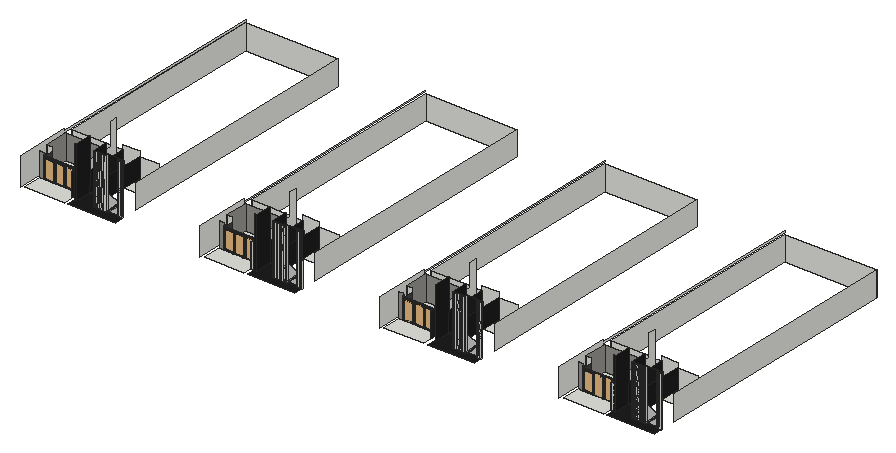
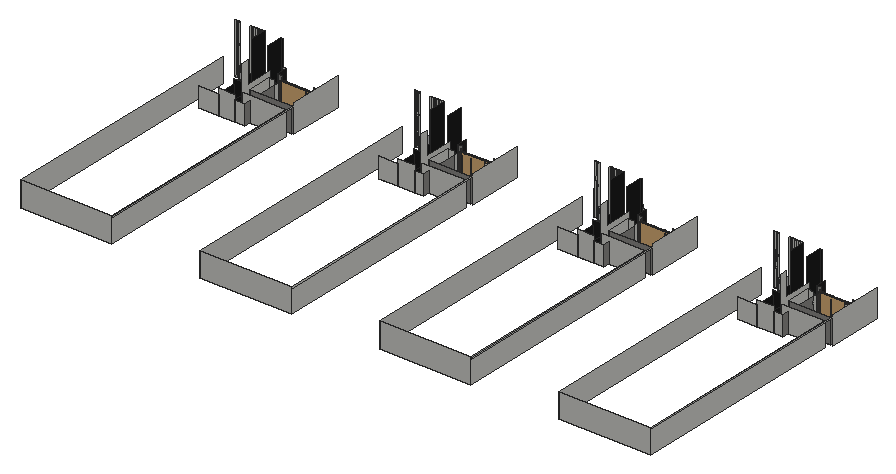
# SketchUp Ruby script. Lengths in inches.
U = 1.inch
M = Sketchup.active_model
def pt(a) = Geom::Point3d.new(a.map { |v| v * U })
def face(e, loops, mat)
  f = e.add_face(loops[0].map { |a| pt(a) })
  loops[1..].each { |l| e.add_face(l.map { |a| pt(a) }).erase! }
  f.material = f.back_material = mat if mat
  f
end
# faces: each face lists its corners as indices into pts; further lists are holes
def faces(e, pts, list, mat = nil) = list.each { |f| face(e, (f[0].is_a?(Array) ? f : [f]).map { |l| l.map { |i| pts[i] } }, mat) }
# xy, xz, yz: faces in a plane at the given z, y or x. An outline is a flat list of corners, or four numbers for a rectangle; further outlines are holes
def ring(l) = l.size == 4 ? [[l[0], l[1]], [l[2], l[1]], [l[2], l[3]], [l[0], l[3]]] : l.each_slice(2).to_a
def flat(e, list, mat, &to3) = list.each { |f| face(e, (f[0].is_a?(Array) ? f : [f]).map { |l| ring(l).map { |u, v| to3.(u, v) } }, mat) }
def xy(e, z, list, mat = nil) = flat(e, list, mat) { |x, y| [x, y, z] }
def xz(e, y, list, mat = nil) = flat(e, list, mat) { |x, z| [x, y, z] }
def yz(e, x, list, mat = nil) = flat(e, list, mat) { |y, z| [x, y, z] }
def lines(e, pts, list) = list.each { |a, b| e.add_line(pt(pts[a]), pt(pts[b])) }
# prism: a flat outline (further loops are holes) pulled along v
def prism(e, loops, v, mat = nil)
  f = face(e, loops, mat); d = Geom::Vector3d.new(v.map { |x| x * U })
  f.pushpull(f.normal.samedirection?(d) ? d.length : -d.length)
end
def box(e, o, s, mat = nil) = prism(e, [[o, [o[0] + s[0], o[1], o[2]], [o[0] + s[0], o[1] + s[1], o[2]], [o[0], o[1] + s[1], o[2]]]], [0, 0, s[2]], mat)
def at(x, y, z, deg = 0) = Geom::Transformation.translation(pt([x, y, z])) * Geom::Transformation.rotation(ORIGIN, Z_AXIS, deg.degrees)
def axes(o, x, y, z) = Geom::Transformation.new([*x, 0, *y, 0, *z, 0, *pt(o).to_a, 1])
def part(name) = M.definitions.add(name)
# library, detail: a bought-in or finely detailed component or shape, given as its bounding box
def library(name, o, s) = part(name).tap { |d| box(d.entities, o, s) }
def detail(e, o, s) = box(e.add_group.entities, o, s)
def put(e, d, t, mat = nil) = e.add_instance(d, t).tap { |i| i.material = mat if mat }
def group(e, t, mat = nil) = e.add_group.tap { |g| g.transformation = t; g.material = mat if mat }.entities
root = M.entities
M.materials.add("Wine2").color = [0, 0, 0]
M.materials["Wine2"].alpha = 0
M.materials.add("[0130_Gainsboro]").color = [39, 45, 50]
M.materials.add("[Carrera Marble]").color = [207, 207, 207]
M.materials.add("[Color M08]").color = [30, 30, 30]
M.materials.add("[Field Square Tile]").color = [211, 167, 108]
M.materials.add("[Granite Dark Gray]").color = [38, 37, 37]
M.materials.add("[Granite Light Gray]").color = [149, 148, 144]
M.materials.add("[Granite Tile]1").color = [68, 65, 63]
M.materials.add("[Slate]").color = [102, 110, 108]
c1 = part("Group\#55")
xy(c1.entities,0,[[0,-0.98,43.07,0],[0,0,43.07,1.4]],"[0130_Gainsboro]")
xy(c1.entities,0.3,[[0.3,-1.43,42.77,-0.98]],"[0130_Gainsboro]")
xy(c1.entities,2.95,[[2.95,-1.43,40.12,-0.63],[2.95,-0.63,40.12,0],[2.95,0,40.12,0.64],[2.95,0.64,40.12,1.4]],"[0130_Gainsboro]")
xy(c1.entities,3.54,[[3.54,-0.63,39.53,0],[3.54,0,39.53,0.64]],"[0130_Gainsboro]")
xy(c1.entities,111.8125,[[3.54,-0.63,39.53,0],[3.54,0,39.53,0.64]],"[0130_Gainsboro]")
xy(c1.entities,112.4,[[2.95,-1.43,40.12,-0.63],[2.95,-0.63,40.12,0],[2.95,0,40.12,0.64],[2.95,0.64,40.12,1.4]],"[0130_Gainsboro]")
xy(c1.entities,115.05,[[0.3,-1.43,42.77,-0.98]],"[0130_Gainsboro]")
xy(c1.entities,115.35,[[0,-0.98,43.07,0],[0,0,43.07,1.4]],"[0130_Gainsboro]")
xz(c1.entities,-1.43,[[[0.3,0.3,42.77,115.05],[2.95,2.95,40.12,112.4]]],"[0130_Gainsboro]")
xz(c1.entities,-0.98,[[[0,0,43.07,115.35],[0.3,0.3,42.77,115.05]]],"[0130_Gainsboro]")
xz(c1.entities,-0.63,[[[2.95,2.95,40.12,112.4],[3.54,3.54,39.53,111.8125]]],"[0130_Gainsboro]")
xz(c1.entities,0,[[3.54,3.54,39.53,111.8125]],"Wine2")
xz(c1.entities,0,[[[0,0,43.07,115.35],[2.95,2.95,40.12,112.4]],[[2.95,2.95,40.12,112.4],[3.54,3.54,39.53,111.8125]]],"[0130_Gainsboro]")
xz(c1.entities,0.64,[[[2.95,2.95,40.12,112.4],[3.54,3.54,39.53,111.8125]]],"[0130_Gainsboro]")
xz(c1.entities,1.4,[[[0,0,43.07,115.35],[2.95,2.95,40.12,112.4]]],"[0130_Gainsboro]")
yz(c1.entities,0,[[-0.98,0,0,115.35],[0,0,1.4,115.35]],"[0130_Gainsboro]")
yz(c1.entities,0.3,[[-1.43,0.3,-0.98,115.05]],"[0130_Gainsboro]")
yz(c1.entities,2.95,[[-1.43,2.95,-0.63,112.4],[-0.63,2.95,0,112.4],[0,2.95,0.64,112.4],[0.64,2.95,1.4,112.4]],"[0130_Gainsboro]")
yz(c1.entities,3.54,[[-0.63,3.54,0,111.8125],[0,3.54,0.64,111.8125]],"[0130_Gainsboro]")
yz(c1.entities,39.53,[[-0.63,3.54,0,111.8125],[0,3.54,0.64,111.8125]],"[0130_Gainsboro]")
yz(c1.entities,40.12,[[-1.43,2.95,-0.63,112.4],[-0.63,2.95,0,112.4],[0,2.95,0.64,112.4],[0.64,2.95,1.4,112.4]],"[0130_Gainsboro]")
yz(c1.entities,42.77,[[-1.43,0.3,-0.98,115.05]],"[0130_Gainsboro]")
yz(c1.entities,43.07,[[-0.98,0,0,115.35],[0,0,1.4,115.35]],"[0130_Gainsboro]")
c2 = part("Component\#21")
put(c2.entities,c1,axes([90.57,1.43,0],[1.05148,0,0],[0,1,0],[0,0,1]))
put(c2.entities,c1,axes([0,1.43,0],[1.05148,0,0],[0,1,0],[0,0,1]))
put(c2.entities,c1,axes([45.29,1.43,0],[1.05148,0,0],[0,1,0],[0,0,1]))
c3 = library("Curtains",[0,0,0],[121.73,8.19,117.22])
xy(root,134.5,[[232.963,2303.93,427.095,2396.678],[1111.713,2303.93,1305.845,2396.678],[1990.463,2303.93,2184.595,2396.678],[2869.213,2303.93,3063.345,2396.678],[252.776,2396.678,406.845,2446.647],
  [1131.526,2396.678,1285.595,2446.647],[2010.276,2396.678,2164.345,2446.647],[2889.026,2396.678,3043.095,2446.647],[406.845,2425.459,406.845,2446.647,433.97,2446.647,433.97,2532.834,444.783,2532.834,444.783,2425.459],[444.783,2425.459,453.702,2532.834],
  [1285.595,2425.459,1285.595,2446.647,1312.72,2446.647,1312.72,2532.834,1323.533,2532.834,1323.533,2425.459],[1323.533,2425.459,1332.452,2532.834],[2164.345,2425.459,2164.345,2446.647,2191.47,2446.647,2191.47,2532.834,2202.283,2532.834,2202.283,2425.459],[2202.283,2425.459,2211.202,2532.834],[3043.095,2425.459,3043.095,2446.647,3070.22,2446.647,3070.22,2532.834,3081.033,2532.834,3081.033,2425.459],
  [3081.033,2425.459,3089.952,2532.834],[228.776,2446.647,406.845,2562.822],[406.845,2446.647,433.97,2532.834],[1107.526,2446.647,1285.595,2562.822],[1285.595,2446.647,1312.72,2532.834],
  [1986.276,2446.647,2164.345,2562.822],[2164.345,2446.647,2191.47,2532.834],[2865.026,2446.647,3043.095,2562.822],[3043.095,2446.647,3070.22,2532.834],[406.845,2532.834,433.97,2562.822],
  [433.97,2532.834,433.97,2562.822,406.845,2562.822,406.845,2597.799,444.783,2597.799,444.783,2532.834],[444.783,2532.834,453.702,2532.834,453.702,2628.146,406.845,2628.146,406.845,2597.799,444.783,2597.799],[534.46,2532.834,629.772,2628.146],[1285.595,2532.834,1312.72,2562.822],[1312.72,2532.834,1312.72,2562.822,1285.595,2562.822,1285.595,2597.799,1323.533,2597.799,1323.533,2532.834],
  [1323.533,2532.834,1332.452,2532.834,1332.452,2628.146,1285.595,2628.146,1285.595,2597.799,1323.533,2597.799],[1413.21,2532.834,1508.522,2628.146],[2164.345,2532.834,2191.47,2562.822],[2191.47,2532.834,2191.47,2562.822,2164.345,2562.822,2164.345,2597.799,2202.283,2597.799,2202.283,2532.834],[2202.283,2532.834,2211.202,2532.834,2211.202,2628.146,2164.345,2628.146,2164.345,2597.799,2202.283,2597.799],
  [2291.96,2532.834,2387.272,2628.146],[3043.095,2532.834,3070.22,2562.822],[3070.22,2532.834,3070.22,2562.822,3043.095,2562.822,3043.095,2597.799,3081.033,2597.799,3081.033,2532.834],[3081.033,2532.834,3089.952,2532.834,3089.952,2628.146,3043.095,2628.146,3043.095,2597.799,3081.033,2597.799],[3170.71,2532.834,3266.022,2628.146]])
xy(root,134.5,[[444.783,2303.93,676.54,2303.93,676.54,2343.959,672.557,2343.959,672.557,2346.709,671.731,2346.709,671.731,2343.959,666.307,2343.959,666.307,2346.709,665.106,2346.709,665.106,2343.959,659.682,2343.959,659.682,2346.709,658.481,2346.709,658.481,2343.959,653.057,2343.959,653.057,2354.271,605.186,2354.271,605.186,2349.146,599.509,2349.146,599.509,2343.959,594.085,2343.959,594.085,2346.709,592.884,2346.709,592.884,2343.959,587.46,2343.959,587.46,2346.709,586.259,2346.709,586.259,2343.959,580.835,2343.959,580.835,2346.709,579.634,2346.709,579.634,2343.959,574.21,2343.959,574.21,2346.709,573.009,2346.709,573.009,2343.959,567.585,2343.959,567.585,2346.709,566.384,2346.709,566.384,2343.959,560.96,2343.959,560.96,2346.709,559.759,2346.709,559.759,2343.959,554.335,2343.959,554.335,2346.709,553.134,2346.709,553.134,2343.959,547.71,2343.959,547.71,2346.709,546.509,2346.709,546.509,2343.959,541.085,2343.959,541.085,2346.709,539.884,2346.709,539.884,2343.959,534.46,2343.959,534.46,2425.459,453.702,2425.459,453.702,2346.709,444.783,2346.709],[1323.533,2303.93,1555.29,2303.93,1555.29,2343.959,1551.307,2343.959,1551.307,2346.709,1550.481,2346.709,1550.481,2343.959,1545.057,2343.959,1545.057,2346.709,1543.856,2346.709,1543.856,2343.959,1538.432,2343.959,1538.432,2346.709,1537.231,2346.709,1537.231,2343.959,1531.807,2343.959,1531.807,2354.271,1483.936,2354.271,1483.936,2349.146,1478.259,2349.146,1478.259,2343.959,1472.835,2343.959,1472.835,2346.709,1471.634,2346.709,1471.634,2343.959,1466.21,2343.959,1466.21,2346.709,1465.009,2346.709,1465.009,2343.959,1459.585,2343.959,1459.585,2346.709,1458.384,2346.709,1458.384,2343.959,1452.96,2343.959,1452.96,2346.709,1451.759,2346.709,1451.759,2343.959,1446.335,2343.959,1446.335,2346.709,1445.134,2346.709,1445.134,2343.959,1439.71,2343.959,1439.71,2346.709,1438.509,2346.709,1438.509,2343.959,1433.085,2343.959,1433.085,2346.709,1431.884,2346.709,1431.884,2343.959,1426.46,2343.959,1426.46,2346.709,1425.259,2346.709,1425.259,2343.959,1419.835,2343.959,1419.835,2346.709,1418.634,2346.709,1418.634,2343.959,1413.21,2343.959,1413.21,2425.459,1332.452,2425.459,1332.452,2346.709,1323.533,2346.709],[2202.283,2303.93,2434.04,2303.93,2434.04,2343.959,2430.057,2343.959,2430.057,2346.709,2429.231,2346.709,2429.231,2343.959,2423.807,2343.959,2423.807,2346.709,2422.606,2346.709,2422.606,2343.959,2417.182,2343.959,2417.182,2346.709,2415.981,2346.709,2415.981,2343.959,2410.557,2343.959,2410.557,2354.271,2362.686,2354.271,2362.686,2349.146,2357.009,2349.146,2357.009,2343.959,2351.585,2343.959,2351.585,2346.709,2350.384,2346.709,2350.384,2343.959,2344.96,2343.959,2344.96,2346.709,2343.759,2346.709,2343.759,2343.959,2338.335,2343.959,2338.335,2346.709,2337.134,2346.709,2337.134,2343.959,2331.71,2343.959,2331.71,2346.709,2330.509,2346.709,2330.509,2343.959,2325.085,2343.959,2325.085,2346.709,2323.884,2346.709,2323.884,2343.959,2318.46,2343.959,2318.46,2346.709,2317.259,2346.709,2317.259,2343.959,2311.835,2343.959,2311.835,2346.709,2310.634,2346.709,2310.634,2343.959,2305.21,2343.959,2305.21,2346.709,2304.009,2346.709,2304.009,2343.959,2298.585,2343.959,2298.585,2346.709,2297.384,2346.709,2297.384,2343.959,2291.96,2343.959,2291.96,2425.459,2211.202,2425.459,2211.202,2346.709,2202.283,2346.709],[3081.033,2303.93,3312.79,2303.93,3312.79,2343.959,3308.807,2343.959,3308.807,2346.709,3307.981,2346.709,3307.981,2343.959,3302.557,2343.959,3302.557,2346.709,3301.356,2346.709,3301.356,2343.959,3295.932,2343.959,3295.932,2346.709,3294.731,2346.709,3294.731,2343.959,3289.307,2343.959,3289.307,2354.271,3241.436,2354.271,3241.436,2349.146,3235.759,2349.146,3235.759,2343.959,3230.335,2343.959,3230.335,2346.709,3229.134,2346.709,3229.134,2343.959,3223.71,2343.959,3223.71,2346.709,3222.509,2346.709,3222.509,2343.959,3217.085,2343.959,3217.085,2346.709,3215.884,2346.709,3215.884,2343.959,3210.46,2343.959,3210.46,2346.709,3209.259,2346.709,3209.259,2343.959,3203.835,2343.959,3203.835,2346.709,3202.634,2346.709,3202.634,2343.959,3197.21,2343.959,3197.21,2346.709,3196.009,2346.709,3196.009,2343.959,3190.585,2343.959,3190.585,2346.709,3189.384,2346.709,3189.384,2343.959,3183.96,2343.959,3183.96,2346.709,3182.759,2346.709,3182.759,2343.959,3177.335,2343.959,3177.335,2346.709,3176.134,2346.709,3176.134,2343.959,3170.71,2343.959,3170.71,2425.459,3089.952,2425.459,3089.952,2346.709,3081.033,2346.709],[453.702,2425.459,534.46,2628.146],
  [1332.452,2425.459,1413.21,2628.146],[2211.202,2425.459,2291.96,2628.146],[3089.952,2425.459,3170.71,2628.146]],"[Color M08]")
xz(root,2346.709,[[534.46,134.5,539.884,380.5],[539.884,134.5,541.085,380.5],[541.085,134.5,546.509,380.5],[546.509,134.5,547.71,380.5],[547.71,134.5,553.134,380.5],
  [553.134,134.5,554.335,380.5],[554.335,134.5,559.759,380.5],[559.759,134.5,560.96,380.5],[560.96,134.5,566.384,380.5],[566.384,134.5,567.585,380.5],
  [567.585,134.5,573.009,380.5],[573.009,134.5,574.21,380.5],[574.21,134.5,579.634,380.5],[579.634,134.5,580.835,380.5],[580.835,134.5,586.259,380.5],
  [586.259,134.5,587.46,380.5],[587.46,134.5,592.884,380.5],[592.884,134.5,594.085,380.5],[594.085,134.5,599.161,380.5],[599.161,134.5,599.509,380.5],
  [653.057,134.5,658.481,380.5],[658.481,134.5,659.682,380.5],[659.682,134.5,665.106,380.5],[665.106,134.5,666.307,380.5],[666.307,134.5,671.731,380.5],
  [671.731,134.5,672.557,380.5],[672.557,134.5,676.54,380.5],[676.54,134.5,677.981,254.5],[1305.845,134.5,1321.095,134.5,1321.095,254.5,1312.72,254.5,1312.72,251.5,1305.845,251.5],[1413.21,134.5,1418.634,380.5],
  [1418.634,134.5,1419.835,380.5],[1419.835,134.5,1425.259,380.5],[1425.259,134.5,1426.46,380.5],[1426.46,134.5,1431.884,380.5],[1431.884,134.5,1433.085,380.5],
  [1433.085,134.5,1438.509,380.5],[1438.509,134.5,1439.71,380.5],[1439.71,134.5,1445.134,380.5],[1445.134,134.5,1446.335,380.5],[1446.335,134.5,1451.759,380.5],
  [1451.759,134.5,1452.96,380.5],[1452.96,134.5,1458.384,380.5],[1458.384,134.5,1459.585,380.5],[1459.585,134.5,1465.009,380.5],[1465.009,134.5,1466.21,380.5],
  [1466.21,134.5,1471.634,380.5],[1471.634,134.5,1472.835,380.5],[1472.835,134.5,1477.911,380.5],[1477.911,134.5,1478.259,380.5],[1531.807,134.5,1537.231,380.5],
  [1537.231,134.5,1538.432,380.5],[1538.432,134.5,1543.856,380.5],[1543.856,134.5,1545.057,380.5],[1545.057,134.5,1550.481,380.5],[1550.481,134.5,1551.307,380.5],
  [1551.307,134.5,1555.29,380.5],[1555.29,134.5,1556.731,254.5],[2298.585,134.5,2304.009,380.5],[2304.009,134.5,2305.21,380.5],[2305.21,134.5,2310.634,380.5],
  [2310.634,134.5,2311.835,380.5],[2311.835,134.5,2317.259,380.5],[2317.259,134.5,2318.46,380.5],[2318.46,134.5,2323.884,380.5],[2323.884,134.5,2325.085,380.5],
  [2325.085,134.5,2330.509,380.5],[2330.509,134.5,2331.71,380.5],[2331.71,134.5,2337.134,380.5],[2337.134,134.5,2338.335,380.5],[2338.335,134.5,2343.759,380.5],
  [2343.759,134.5,2344.96,380.5],[2344.96,134.5,2350.384,380.5],[2351.585,134.5,2356.661,380.5],[2356.661,134.5,2357.009,380.5],[2410.557,134.5,2415.981,380.5],
  [2415.981,134.5,2417.182,380.5],[2417.182,134.5,2422.606,380.5],[2422.606,134.5,2423.807,380.5],[2423.807,134.5,2429.231,380.5],[2429.231,134.5,2430.057,380.5],
  [2430.057,134.5,2434.04,380.5],[2434.04,134.5,2435.481,254.5],[3063.345,134.5,3078.595,134.5,3078.595,254.5,3070.22,254.5,3070.22,251.5,3063.345,251.5],[3170.71,134.5,3176.134,380.5],[3176.134,134.5,3177.335,380.5],
  [3177.335,134.5,3182.759,380.5],[3182.759,134.5,3183.96,380.5],[3183.96,134.5,3189.384,380.5],[3189.384,134.5,3190.585,380.5],[3190.585,134.5,3196.009,380.5],
  [3196.009,134.5,3197.21,380.5],[3197.21,134.5,3202.634,380.5],[3202.634,134.5,3203.835,380.5],[3203.835,134.5,3209.259,380.5],[3209.259,134.5,3210.46,380.5],
  [3210.46,134.5,3215.884,380.5],[3215.884,134.5,3217.085,380.5],[3217.085,134.5,3222.509,380.5],[3222.509,134.5,3223.71,380.5],[3223.71,134.5,3229.134,380.5],
  [3229.134,134.5,3230.335,380.5],[3230.335,134.5,3235.411,380.5],[3235.411,134.5,3235.759,380.5],[3289.307,134.5,3294.731,380.5],[3294.731,134.5,3295.932,380.5],
  [3295.932,134.5,3301.356,380.5],[3301.356,134.5,3302.557,380.5],[3302.557,134.5,3307.981,380.5],[3307.981,134.5,3308.807,380.5],[3308.807,134.5,3312.79,380.5],
  [3312.79,134.5,3314.231,254.5]])
xz(root,2346.709,[[442.345,134.5,453.702,134.5,453.702,380.5,444.783,380.5,444.783,270.8125,442.345,270.8125],[1321.095,134.5,1332.452,134.5,1332.452,380.5,1323.533,380.5,1323.533,270.8125,1321.095,270.8125],[3078.595,134.5,3089.952,134.5,3089.952,380.5,3081.033,380.5,3081.033,270.8125,3078.595,270.8125]],"[Color M08]")
xz(root,2349.146,[[599.509,134.5,605.186,134.5,653.057,178.842,653.057,188.267],[1478.259,134.5,1483.936,134.5,1531.807,178.842,1531.807,188.267],[2357.009,134.5,2362.686,134.5,2410.557,178.842,2410.557,188.267],[3235.759,134.5,3241.436,134.5,3289.307,178.842,3289.307,188.267]],"[Field Square Tile]")
xz(root,2354.271,[[599.509,134.5,653.057,188.267,599.509,215.747],[605.186,134.5,653.057,134.5,653.057,178.842],[1478.259,134.5,1531.807,188.267,1478.259,215.747],[1483.936,134.5,1531.807,134.5,1531.807,178.842],[2357.009,134.5,2410.557,188.267,2357.009,215.747],
  [2362.686,134.5,2410.557,134.5,2410.557,178.842],[3235.759,134.5,3289.307,188.267,3235.759,215.747],[3241.436,134.5,3289.307,134.5,3289.307,178.842]],"[Carrera Marble]")
xz(root,2396.678,[[232.963,134.5,252.776,251.5],[406.845,134.5,427.095,251.5],[1111.713,134.5,1131.526,251.5],[1285.595,134.5,1305.845,251.5],[1990.463,134.5,2010.276,251.5],
  [2164.345,134.5,2184.595,251.5],[2869.213,134.5,2889.026,251.5],[3043.095,134.5,3063.345,251.5]],"[Granite Light Gray]")
xz(root,2425.459,[[406.845,134.5,444.783,231],[444.783,134.5,453.702,231],[1285.595,134.5,1323.533,231],[1323.533,134.5,1332.452,231],[2164.345,134.5,2202.283,231],
  [2202.283,134.5,2211.202,231],[3043.095,134.5,3081.033,231],[3081.033,134.5,3089.952,231]])
xz(root,2446.647,[[228.776,134.5,252.776,254.5],[406.845,134.5,433.97,254.5],[1107.526,134.5,1131.526,254.5],[1285.595,134.5,1312.72,254.5],[1986.276,134.5,2010.276,254.5],
  [2164.345,134.5,2191.47,254.5],[2865.026,134.5,2889.026,254.5],[3043.095,134.5,3070.22,254.5]])
xz(root,2532.834,[[453.702,134.5,534.46,254.5],[1332.452,134.5,1413.21,254.5],[2211.202,134.5,2291.96,254.5],[3089.952,134.5,3170.71,254.5]],"[Color M08]")
xz(root,2562.822,[[228.776,134.5,433.97,254.5],[1107.526,134.5,1312.72,254.5],[1986.276,134.5,2191.47,254.5],[2865.026,134.5,3070.22,254.5]],"[Granite Light Gray]")
xz(root,2597.799,[[228.776,134.5,444.783,254.5],[1107.526,134.5,1323.533,254.5],[1986.276,134.5,2202.283,254.5],[2865.026,134.5,3081.033,254.5]])
xz(root,2628.146,[[406.845,134.5,453.702,231],[453.702,134.5,534.46,254.5],[534.46,134.5,629.772,231],[1285.595,134.5,1332.452,231],[1332.452,134.5,1413.21,254.5],
  [1413.21,134.5,1508.522,231],[2164.345,134.5,2211.202,231],[2211.202,134.5,2291.96,254.5],[2291.96,134.5,2387.272,231],[3043.095,134.5,3089.952,231],
  [3089.952,134.5,3170.71,254.5],[3170.71,134.5,3266.022,231]])
xz(root,3661.445,[[228.776,134.5,676.54,254.5],[1107.526,134.5,1555.29,254.5],[1986.276,134.5,2434.04,254.5],[2865.026,134.5,3312.79,254.5]])
yz(root,218.97,[[2294.125,134.5,2294.125,270.8125,2562.822,270.8125,2562.822,260.5,3671.25,260.5,3671.25,254.5,2562.822,254.5,2562.822,134.5]])
yz(root,228.776,[[2597.799,134.5,3661.445,254.5]])
yz(root,228.776,[[2446.647,134.5,2562.822,254.5]],"[Granite Light Gray]")
yz(root,252.776,[[2396.678,134.5,2446.647,134.5,2446.647,230.894,2402.303,230.894,2402.303,241.519,2396.678,241.519]],"[Granite Tile]1")
yz(root,406.845,[[2425.459,134.5,2446.647,230.894]])
yz(root,406.845,[[2446.647,134.5,2628.146,231]],"[Granite Light Gray]")
yz(root,406.845,[[2396.678,134.5,2396.678,240.932,2399.776,241.17,2399.81,241.167,2399.809,241.173,2401.365,241.293,2401.365,240.89,2402.303,240.89,2402.303,230.894,2425.459,230.894,2425.459,134.5]],"[Granite Tile]1")
yz(root,427.095,[[2346.709,134.5,2396.678,251.5]],"[Granite Dark Gray]")
yz(root,433.97,[[2446.647,134.5,2562.822,254.5]])
yz(root,444.783,[[2425.459,134.5,2597.799,134.5,2597.799,380.5,2562.822,380.5,2562.822,270.8125,2425.459,270.8125]])
yz(root,453.702,[[2346.709,134.5,2425.459,380.5],[2425.459,134.5,2628.146,231]],"[Color M08]")
yz(root,534.46,[[2346.709,134.5,2425.459,380.5],[2425.459,134.5,2628.146,231]],"[Color M08]")
yz(root,599.509,[[2346.709,134.5,2354.271,380.5]])
yz(root,653.057,[[2346.709,134.5,2346.709,380.5,2349.146,380.5,2349.146,374.002,2354.271,374.002,2354.271,290.711,2349.146,290.711,2349.146,275.136,2354.271,275.136,2354.271,192.888,2349.146,192.888,2349.146,178.842,2354.271,178.842,2354.271,134.5]])
yz(root,676.54,[[2425.459,134.5,3661.445,254.5]])
yz(root,1097.72,[[2294.125,134.5,2294.125,270.8125,2562.822,270.8125,2562.822,260.5,3671.25,260.5,3671.25,254.5,2562.822,254.5,2562.822,134.5]])
yz(root,1107.526,[[2597.799,134.5,3661.445,254.5]])
yz(root,1107.526,[[2446.647,134.5,2562.822,254.5]],"[Granite Light Gray]")
yz(root,1131.526,[[2396.678,134.5,2446.647,134.5,2446.647,230.894,2402.303,230.894,2402.303,241.519,2396.678,241.519]],"[Granite Tile]1")
yz(root,1285.595,[[2425.459,134.5,2446.647,230.894]])
yz(root,1285.595,[[2446.647,134.5,2628.146,231]],"[Granite Light Gray]")
yz(root,1285.595,[[2396.678,134.5,2396.678,240.932,2399.776,241.17,2399.81,241.167,2399.809,241.173,2401.365,241.293,2401.365,240.89,2402.303,240.89,2402.303,230.894,2425.459,230.894,2425.459,134.5]],"[Granite Tile]1")
yz(root,1305.845,[[2346.709,134.5,2396.678,251.5]],"[Granite Dark Gray]")
yz(root,1312.72,[[2446.647,134.5,2562.822,254.5]])
yz(root,1323.533,[[2425.459,134.5,2597.799,134.5,2597.799,380.5,2562.822,380.5,2562.822,270.8125,2425.459,270.8125]])
yz(root,1332.452,[[2346.709,134.5,2425.459,380.5],[2425.459,134.5,2628.146,231]],"[Color M08]")
yz(root,1413.21,[[2346.709,134.5,2425.459,380.5],[2425.459,134.5,2628.146,231]],"[Color M08]")
yz(root,1478.259,[[2346.709,134.5,2354.271,380.5]])
yz(root,1531.807,[[2346.709,134.5,2346.709,380.5,2349.146,380.5,2349.146,374.002,2354.271,374.002,2354.271,290.711,2349.146,290.711,2349.146,275.136,2354.271,275.136,2354.271,192.888,2349.146,192.888,2349.146,178.842,2354.271,178.842,2354.271,134.5]])
yz(root,1555.29,[[2425.459,134.5,3661.445,254.5]])
yz(root,1976.47,[[2294.125,134.5,2294.125,270.8125,2562.822,270.8125,2562.822,260.5,3671.25,260.5,3671.25,254.5,2562.822,254.5,2562.822,134.5]])
yz(root,1986.276,[[2597.799,134.5,3661.445,254.5]])
yz(root,1986.276,[[2446.647,134.5,2562.822,254.5]],"[Granite Light Gray]")
yz(root,2010.276,[[2396.678,134.5,2446.647,134.5,2446.647,230.894,2402.303,230.894,2402.303,241.519,2396.678,241.519]],"[Granite Tile]1")
yz(root,2164.345,[[2425.459,134.5,2446.647,230.894]])
yz(root,2164.345,[[2446.647,134.5,2628.146,231]],"[Granite Light Gray]")
yz(root,2164.345,[[2396.678,134.5,2396.678,240.932,2399.776,241.17,2399.81,241.167,2399.809,241.173,2401.365,241.293,2401.365,240.89,2402.303,240.89,2402.303,230.894,2425.459,230.894,2425.459,134.5]],"[Granite Tile]1")
yz(root,2184.595,[[2346.709,134.5,2396.678,251.5]],"[Granite Dark Gray]")
yz(root,2191.47,[[2446.647,134.5,2562.822,254.5]])
yz(root,2202.283,[[2425.459,134.5,2597.799,134.5,2597.799,380.5,2562.822,380.5,2562.822,270.8125,2425.459,270.8125]])
yz(root,2211.202,[[2346.709,134.5,2425.459,380.5],[2425.459,134.5,2628.146,231]],"[Color M08]")
yz(root,2291.96,[[2346.709,134.5,2425.459,380.5],[2425.459,134.5,2628.146,231]],"[Color M08]")
yz(root,2357.009,[[2346.709,134.5,2354.271,380.5]])
yz(root,2410.557,[[2346.709,134.5,2346.709,380.5,2349.146,380.5,2349.146,374.002,2354.271,374.002,2354.271,290.711,2349.146,290.711,2349.146,275.136,2354.271,275.136,2354.271,192.888,2349.146,192.888,2349.146,178.842,2354.271,178.842,2354.271,134.5]])
yz(root,2434.04,[[2425.459,134.5,3661.445,254.5]])
yz(root,2855.22,[[2294.125,134.5,2294.125,270.8125,2562.822,270.8125,2562.822,260.5,3671.25,260.5,3671.25,254.5,2562.822,254.5,2562.822,134.5]])
yz(root,2865.026,[[2597.799,134.5,3661.445,254.5]])
yz(root,2865.026,[[2446.647,134.5,2562.822,254.5]],"[Granite Light Gray]")
yz(root,2889.026,[[2396.678,134.5,2446.647,134.5,2446.647,230.894,2402.303,230.894,2402.303,241.519,2396.678,241.519]],"[Granite Tile]1")
yz(root,3043.095,[[2425.459,134.5,2446.647,230.894]])
yz(root,3043.095,[[2446.647,134.5,2628.146,231]],"[Granite Light Gray]")
yz(root,3043.095,[[2396.678,134.5,2396.678,240.932,2399.776,241.17,2399.81,241.167,2399.809,241.173,2401.365,241.293,2401.365,240.89,2402.303,240.89,2402.303,230.894,2425.459,230.894,2425.459,134.5]],"[Granite Tile]1")
yz(root,3063.345,[[2346.709,134.5,2396.678,251.5]],"[Granite Dark Gray]")
yz(root,3070.22,[[2446.647,134.5,2562.822,254.5]])
yz(root,3081.033,[[2425.459,134.5,2597.799,134.5,2597.799,380.5,2562.822,380.5,2562.822,270.8125,2425.459,270.8125]])
yz(root,3089.952,[[2346.709,134.5,2425.459,380.5],[2425.459,134.5,2628.146,231]],"[Color M08]")
yz(root,3170.71,[[2346.709,134.5,2425.459,380.5],[2425.459,134.5,2628.146,231]],"[Color M08]")
yz(root,3235.759,[[2346.709,134.5,2354.271,380.5]])
yz(root,3289.307,[[2346.709,134.5,2346.709,380.5,2349.146,380.5,2349.146,374.002,2354.271,374.002,2354.271,290.711,2349.146,290.711,2349.146,275.136,2354.271,275.136,2354.271,192.888,2349.146,192.888,2349.146,178.842,2354.271,178.842,2354.271,134.5]])
yz(root,3312.79,[[2425.459,134.5,3661.445,254.5]])
p = [[653.057,2354.271,188.267],[599.509,2354.271,134.5],[599.509,2349.146,134.5],[653.057,2349.146,188.267],[605.186,2354.271,134.5],[653.057,2354.271,178.842],
  [653.057,2349.146,178.842],[605.186,2349.146,134.5],[1531.807,2354.271,188.267],[1478.259,2354.271,134.5],[1478.259,2349.146,134.5],[1531.807,2349.146,188.267],
  [1483.936,2354.271,134.5],[1531.807,2354.271,178.842],[1531.807,2349.146,178.842],[1483.936,2349.146,134.5],[2410.557,2354.271,188.267],[2357.009,2354.271,134.5],
  [2357.009,2349.146,134.5],[2410.557,2349.146,188.267],[2362.686,2354.271,134.5],[2410.557,2354.271,178.842],[2410.557,2349.146,178.842],[2362.686,2349.146,134.5],
  [3289.307,2354.271,188.267],[3235.759,2354.271,134.5],[3235.759,2349.146,134.5],[3289.307,2349.146,188.267],[3241.436,2354.271,134.5],[3289.307,2354.271,178.842],
  [3289.307,2349.146,178.842],[3241.436,2349.146,134.5]]
faces(root,p,[[0,1,2,3],[4,5,6,7],[8,9,10,11],[12,13,14,15],[16,17,18,19],[20,21,22,23],[24,25,26,27],[28,29,30,31]])
put(root,c2,axes([2010.28,2396.68,134.5],[1.13,0,0],[0,1,0],[0,0,0.83]))
put(root,c2,axes([252.78,2396.68,134.5],[1.13,0,0],[0,1,0],[0,0,0.83]))
put(root,c2,axes([1131.53,2396.68,134.5],[1.13,0,0],[0,1,0],[0,0,0.83]))
put(root,c2,axes([2889.03,2396.68,134.5],[1.13,0,0],[0,1,0],[0,0,0.83]))
put(root,c3,axes([252.78,2396.68,134.75],[1.29555,0,0],[0,1,0],[0,0,0.8242]),"[Slate]")
put(root,c3,axes([1131.53,2396.68,134.75],[1.29555,0,0],[0,1,0],[0,0,0.8242]),"[Slate]")
put(root,c3,axes([2889.03,2396.68,134.75],[1.29555,0,0],[0,1,0],[0,0,0.8242]),"[Slate]")
put(root,c3,axes([2010.28,2396.68,134.75],[1.29555,0,0],[0,1,0],[0,0,0.8242]),"[Slate]")
